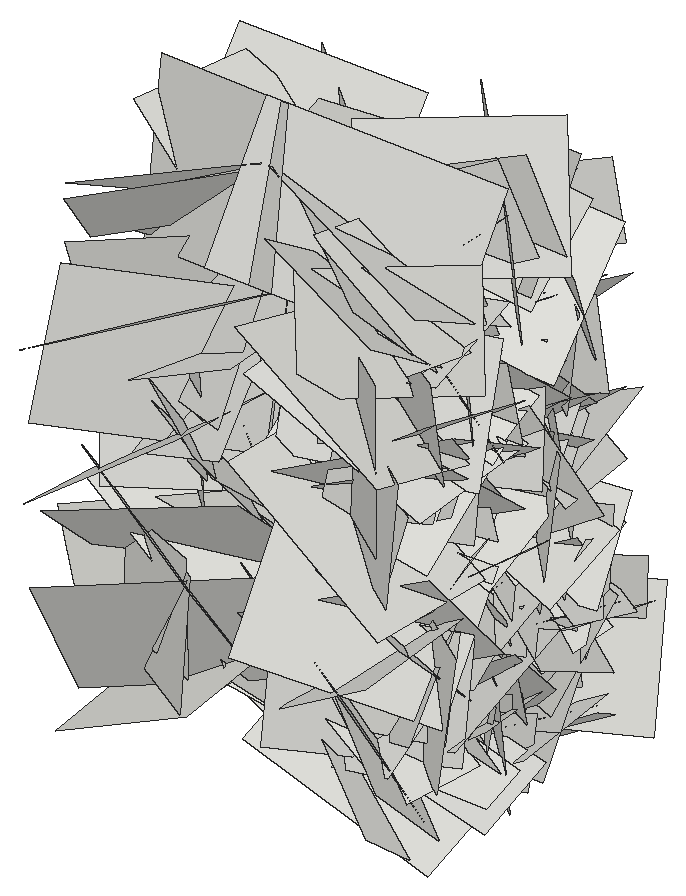
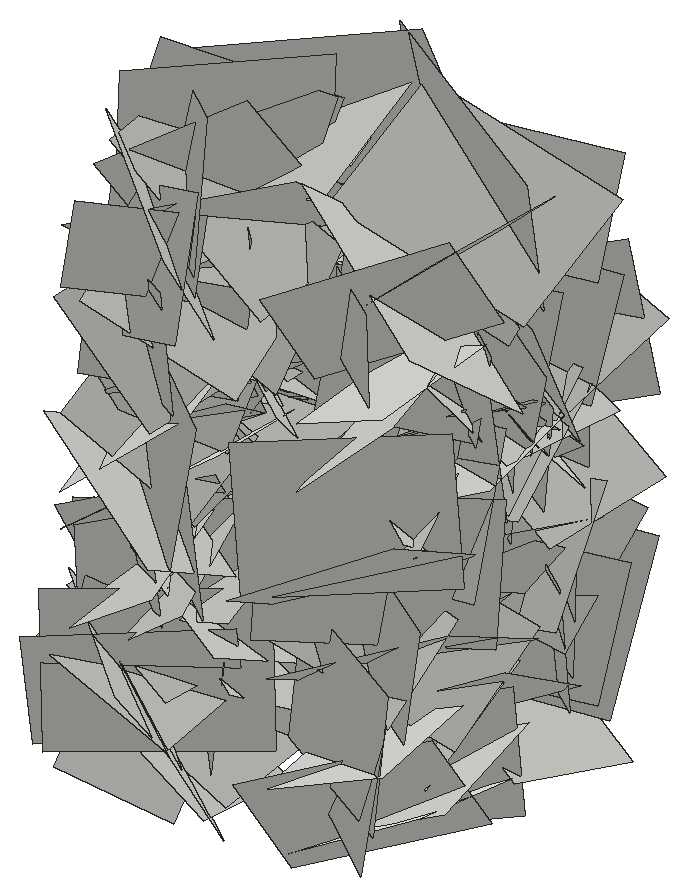
# SketchUp Ruby script. Lengths in inches.
U = 1.inch
M = Sketchup.active_model
def pt(a) = Geom::Point3d.new(a.map { |v| v * U })
def face(e, loops, mat)
  f = e.add_face(loops[0].map { |a| pt(a) })
  loops[1..].each { |l| e.add_face(l.map { |a| pt(a) }).erase! }
  f.material = f.back_material = mat if mat
  f
end
# faces: each face lists its corners as indices into pts; further lists are holes
def faces(e, pts, list, mat = nil) = list.each { |f| face(e, (f[0].is_a?(Array) ? f : [f]).map { |l| l.map { |i| pts[i] } }, mat) }
# xy, xz, yz: faces in a plane at the given z, y or x. An outline is a flat list of corners, or four numbers for a rectangle; further outlines are holes
def ring(l) = l.size == 4 ? [[l[0], l[1]], [l[2], l[1]], [l[2], l[3]], [l[0], l[3]]] : l.each_slice(2).to_a
def flat(e, list, mat, &to3) = list.each { |f| face(e, (f[0].is_a?(Array) ? f : [f]).map { |l| ring(l).map { |u, v| to3.(u, v) } }, mat) }
def xy(e, z, list, mat = nil) = flat(e, list, mat) { |x, y| [x, y, z] }
def xz(e, y, list, mat = nil) = flat(e, list, mat) { |x, z| [x, y, z] }
def yz(e, x, list, mat = nil) = flat(e, list, mat) { |y, z| [x, y, z] }
def lines(e, pts, list) = list.each { |a, b| e.add_line(pt(pts[a]), pt(pts[b])) }
# prism: a flat outline (further loops are holes) pulled along v
def prism(e, loops, v, mat = nil)
  f = face(e, loops, mat); d = Geom::Vector3d.new(v.map { |x| x * U })
  f.pushpull(f.normal.samedirection?(d) ? d.length : -d.length)
end
def box(e, o, s, mat = nil) = prism(e, [[o, [o[0] + s[0], o[1], o[2]], [o[0] + s[0], o[1] + s[1], o[2]], [o[0], o[1] + s[1], o[2]]]], [0, 0, s[2]], mat)
def at(x, y, z, deg = 0) = Geom::Transformation.translation(pt([x, y, z])) * Geom::Transformation.rotation(ORIGIN, Z_AXIS, deg.degrees)
def axes(o, x, y, z) = Geom::Transformation.new([*x, 0, *y, 0, *z, 0, *pt(o).to_a, 1])
def part(name) = M.definitions.add(name)
# library, detail: a bought-in or finely detailed component or shape, given as its bounding box
def library(name, o, s) = part(name).tap { |d| box(d.entities, o, s) }
def detail(e, o, s) = box(e.add_group.entities, o, s)
def put(e, d, t, mat = nil) = e.add_instance(d, t).tap { |i| i.material = mat if mat }
def group(e, t, mat = nil) = e.add_group.tap { |g| g.transformation = t; g.material = mat if mat }.entities
root = M.entities
c1 = part("Component\#6")
p = [[0.01,0,0],[0,3.24,4.54],[4.32,3.24,4.54],[4.33,0,0]]
faces(c1.entities,p,[[0,1,2,3]])
put(root,c1,axes([14.53,139.9,15.42],[0.08068,-0.00169,-0.87701],[0.08263,-0.87681,0.00845],[0.92595,0.07839,0.07566]))
put(root,c1,axes([18.5,139.99,14.29],[-0.01199,-0.16574,0.68191],[0.09091,0.67656,0.16586],[-0.73829,0.086,0.00935]))
put(root,c1,axes([18.5,147.58,14.43],[0.15626,-0.88067,0.15465],[0.14549,0.17716,0.87807],[-0.93656,-0.11942,0.1622]))
put(root,c1,axes([18.5,138.3,10.21],[0.07821,-0.14386,0.79141],[0.12147,0.78851,0.13265],[-0.84394,0.10016,0.09244]))
put(root,c1,axes([14.53,142.2,15.72],[-0.2001,0.61396,-1.10583],[-0.10306,-1.12181,-0.60624],[1.33676,0.00542,-0.21228]))
put(root,c1,axes([14.53,141.25,1.55],[0.11713,-0.0063,1.0149],[-0.13715,1.01248,0.02037],[1.06704,0.13083,-0.10878]))
put(root,c1,axes([14.53,144.34,6.82],[-0.01542,0.93301,-0.17325],[0.14993,-0.1692,-0.92309],[0.99466,0.03997,0.13646]))
put(root,c1,axes([14.53,137.99,14.66],[-0.08461,-0.27233,0.9902],[0.1352,0.98287,0.28059],[1.08015,-0.14435,0.04245]))
put(root,c1,axes([14.53,142.29,19.52],[0.02505,0.60517,0.90894],[-0.1077,0.90642,-0.60085],[1.15246,0.07156,-0.07591]))
put(root,c1,axes([14.53,144.58,9.97],[0.16827,0.58944,-0.69808],[-0.0398,-0.70373,-0.60275],[0.96765,-0.13145,0.0966]))
put(root,c1,axes([18.5,139.8125,20.98],[-0.02151,0.52563,-0.34386],[0.05265,-0.34162,-0.52514],[-0.66372,-0.04413,-0.03051]))
put(root,c1,axes([18.5,142.6,14.22],[0.18899,-0.6396,-0.42028],[-0.00285,-0.43205,0.65638],[-0.81124,-0.14749,-0.10022]))
put(root,c1,axes([18.5,145.36,10.15],[0.14636,-0.64891,0.3527],[0.01811,0.36152,0.65845],[-0.78267,-0.11298,0.08119]))
put(root,c1,axes([18.5,145.42,18.19],[0.07853,-0.05807,0.70782],[0.06912,0.70921,0.05136],[-0.74963,0.05931,0.07889]))
put(root,c1,axes([14.53,146.45,10.34],[0.10559,0.05407,-0.92917],[0.0532,-0.93343,-0.04894],[0.98516,0.04461,0.10223]))
put(root,c1,axes([18.5,141.95,12.73],[0.09992,0.55515,0.3498],[-0.02862,0.35638,-0.5583],[-0.69495,0.06514,0.07329]))
put(root,c1,axes([14.53,137.63,3.85],[-0.23328,-0.07655,1.22947],[0.08564,1.24535,0.092],[1.30295,-0.09556,0.21407]))
put(root,c1,axes([18.5,139.18,13.74],[0.11062,-0.13563,-0.63299],[-0.03095,-0.6415,0.13263],[-0.6855,0.00708,-0.10814]))
put(root,c1,axes([14.53,141.92,3.18],[0.02887,1.0089,0.10446],[0.06921,0.10254,-1.00735],[1.07292,-0.03376,0.06217]))
put(root,c1,axes([14.53,138.34,13.4],[0.1901,0.66514,0.65147],[-0.02496,0.66648,-0.67398],[0.98658,-0.1113,-0.14258]))
put(root,c1,axes([14.53,138.76,9.15],[0.08107,-0.07376,-0.93469],[0.12107,-0.93007,0.08274],[0.98644,0.12021,0.06666]))
put(root,c1,axes([14.53,139.52,8.83],[0.01584,-0.12995,-1.07448],[0.00128,-1.07458,0.12998],[1.14724,0.003,0.01469]))
put(root,c1,axes([14.53,137.41,10.49],[0.17918,0.96529,0.20208],[-0.06958,0.21558,-0.97489],[1.04307,-0.15144,-0.09975]))
put(root,c1,axes([14.53,141.07,4.77],[-0.0925,1.07709,-0.24358],[0.13853,-0.23255,-1.07513],[1.16232,0.11343,0.10875]))
put(root,c1,axes([14.53,143.54,11.83],[-0.01207,0.98557,0.48784],[0.03058,0.48797,-0.98515],[1.16528,-0.0026,0.03091]))
put(root,c1,axes([18.5,142.82,6.12],[-0.04161,-0.60559,-0.03198],[0.13563,-0.03959,0.59276],[-0.62835,0.03156,0.13006]))
put(root,c1,axes([14.53,142.72,8.07],[-0.13823,0.05764,1.30603],[-0.0986,1.30878,-0.06705],[1.38223,0.09912,0.12583]))
put(root,c1,axes([14.53,138.64,15.1],[-0.05154,1.07135,-0.23626],[0.10153,-0.23144,-1.06922],[1.15847,0.06794,0.08319]))
put(root,c1,axes([14.53,138.49,4.97],[-0.13436,1.04009,0.6085],[0.04809,0.61554,-1.04268],[1.27641,0.08629,0.10334]))
put(root,c1,axes([18.5,137.29,3.46],[0.14224,0.61257,0.15159],[-0.04066,0.16261,-0.62315],[-0.66768,0.1206,0.07024]))
put(root,c1,axes([14.53,137.21,11.6875],[-0.11385,0.72886,-0.88593],[0.14818,-0.87485,-0.7367],[1.20699,0.17615,0.00688]))
put(root,c1,axes([14.53,143.17,19.13],[0.20193,0.9279,-0.28366],[0.04691,-0.29708,-0.94209],[1.02744,-0.16881,0.09877]))
put(root,c1,axes([14.53,142.88,1.98],[0.0351,0.64216,0.95117],[0.00533,0.95147,-0.64254],[1.21649,-0.02269,-0.02463]))
put(root,c1,axes([14.53,137.64,18.89],[0.26376,-0.64139,0.69016],[0.02251,0.71746,0.65911],[0.99845,0.15326,-0.19718]))
put(root,c1,axes([14.53,140.93,18.6875],[-0.10901,-0.41314,-1.06231],[0.28274,-1.04573,0.38087],[1.17466,0.21337,-0.19026]))
put(root,c1,axes([14.53,141.75,2.91],[-0.11729,-1.19784,-0.30033],[0.11289,-0.30967,1.19584],[1.30414,-0.08092,-0.13053]))
put(root,c1,axes([14.53,143.08,17.68],[-0.06532,-0.13436,-1.17102],[0.13166,-1.16683,0.12734],[1.24247,0.11658,-0.07506]))
put(root,c1,axes([14.53,140.04,10.48],[-0.03722,-1.27767,0.05021],[-0.04996,0.05148,1.27723],[1.35446,-0.03321,0.04849]))
put(root,c1,axes([14.53,140.59,7.56],[-0.03383,1.06332,0.50099],[0.10932,0.50178,-1.05842],[1.24115,-0.01522,0.10688]))
put(root,c1,axes([14.53,137.94,15.45],[-0.03401,0.89045,-0.73196],[0.17038,-0.72163,-0.88493],[1.2099,0.12665,0.10405]))
put(root,c1,axes([14.53,146.96,20.2],[-0.19126,-1.0536,-0.82739],[0.10265,-0.84293,1.05228],[1.41631,-0.08119,-0.188]))
put(root,c1,axes([14.53,139.77,22.87],[0.12093,1.26112,-0.05281],[-0.18505,-0.03675,-1.25475],[1.32509,-0.12022,-0.17041]))
put(root,c1,axes([14.53,139.44,14.86],[-0.04621,-1.16691,0.31838],[0.12643,0.31289,1.16311],[1.27589,-0.07327,-0.10372]))
put(root,c1,axes([14.53,141.48,7.17],[0.20337,0.82379,-0.77749],[-0.08888,-0.77608,-0.84298],[1.19742,-0.19752,0.06948]))
put(root,c1,axes([14.53,138.37,16.22],[0.07456,0.76169,-0.90937],[0.0504,-0.91204,-0.76025],[1.25638,-0.00862,0.08446]))
put(root,c1,axes([14.53,148.05,8.79],[0.07068,0.0827,-1.14811],[0.1221,-1.14474,-0.07576],[1.21402,0.11031,0.07447]))
put(root,c1,axes([14.53,144.3,10.94],[0.16969,-0.07735,1.18237],[-0.06112,1.19119,0.08573],[1.2545,0.0685,-0.15576]))
put(root,c1,axes([14.53,144.73,5.33],[0.04426,-1.02294,0.56209],[0.16257,0.56238,1.01208],[1.2265,-0.03763,-0.15444]))
put(root,c1,axes([14.53,141.11,14.91],[0.10517,-0.78429,-0.79452],[0.18451,-0.77703,0.78876],[1.16892,0.19321,-0.05302]))
put(root,c1,axes([14.53,134.59,13.6],[0.14779,0.17555,1.29716],[-0.16453,1.29751,-0.15892],[1.37773,0.13612,-0.15813]))
put(root,c1,axes([14.53,148.13,7.79],[0.13698,0.11741,-1.23467],[-0.05668,-1.23967,-0.12348],[1.31343,-0.06574,0.12344]))
put(root,c1,axes([14.53,139.3125,6.46],[-0.05297,-0.89114,0.82127],[0.332,0.78454,0.87035],[1.24093,-0.24794,-0.1978]))
put(root,c1,axes([14.53,142.16,14.375],[-0.02255,-1.26636,-0.09652],[0.2141,-0.09868,1.25016],[1.3291,-0.00559,-0.20302]))
put(root,c1,axes([14.53,141.32,18.93],[-0.00931,-1.12138,0.55372],[0.26786,0.54072,1.09906],[1.29833,-0.1196,-0.22278]))
put(root,c1,axes([14.53,140.96,14.21],[0.1647,-0.56811,1.02456],[0.16232,1.03452,0.5504],[1.23116,-0.0604,-0.20963]))
put(root,c1,axes([14.53,137.06,3.09],[0.11239,-0.69918,1.17187],[0.18512,1.17269,0.68387],[1.43458,-0.09655,-0.18006]))
put(root,c1,axes([14.53,141.18,23.91],[0.20239,-0.45291,-1.29893],[0.24414,-1.28235,0.48098],[1.43758,0.28153,0.10118]))
put(root,c1,axes([28.31,141.18,23.91],[-0.20239,-0.45291,-1.29893],[-0.24414,-1.28235,0.48098],[-1.43758,0.28153,0.10118]))
put(root,c1,axes([28.31,137.06,3.09],[-0.11239,-0.69918,1.17187],[-0.18512,1.17269,0.68387],[-1.43458,-0.09655,-0.18006]))
put(root,c1,axes([28.31,140.96,14.21],[-0.1647,-0.56811,1.02456],[-0.16232,1.03452,0.5504],[-1.23116,-0.0604,-0.20963]))
put(root,c1,axes([28.31,141.32,18.93],[0.00931,-1.12138,0.55372],[-0.26786,0.54072,1.09906],[-1.29833,-0.1196,-0.22278]))
put(root,c1,axes([28.31,142.16,14.375],[0.02255,-1.26636,-0.09652],[-0.2141,-0.09868,1.25016],[-1.3291,-0.00559,-0.20302]))
put(root,c1,axes([28.31,139.3125,6.46],[0.05297,-0.89114,0.82127],[-0.332,0.78454,0.87035],[-1.24093,-0.24794,-0.1978]))
put(root,c1,axes([28.31,148.13,7.79],[-0.13698,0.11741,-1.23467],[0.05668,-1.23967,-0.12348],[-1.31343,-0.06574,0.12344]))
put(root,c1,axes([28.31,134.59,13.6],[-0.14779,0.17555,1.29716],[0.16453,1.29751,-0.15892],[-1.37773,0.13612,-0.15813]))
put(root,c1,axes([28.31,141.11,14.91],[-0.10517,-0.78429,-0.79452],[-0.18451,-0.77703,0.78876],[-1.16892,0.19321,-0.05302]))
put(root,c1,axes([28.31,144.73,5.33],[-0.04426,-1.02294,0.56209],[-0.16257,0.56238,1.01208],[-1.2265,-0.03763,-0.15444]))
put(root,c1,axes([28.31,144.3,10.94],[-0.16969,-0.07735,1.18237],[0.06112,1.19119,0.08573],[-1.2545,0.0685,-0.15576]))
put(root,c1,axes([28.31,138.37,16.22],[-0.07456,0.76169,-0.90937],[-0.0504,-0.91204,-0.76025],[-1.25638,-0.00862,0.08446]))
put(root,c1,axes([28.31,141.48,7.17],[-0.20337,0.82379,-0.77749],[0.08888,-0.77608,-0.84298],[-1.19742,-0.19752,0.06948]))
put(root,c1,axes([28.31,139.44,14.86],[0.04621,-1.16691,0.31838],[-0.12643,0.31289,1.16311],[-1.27589,-0.07327,-0.10372]))
put(root,c1,axes([28.31,139.77,22.87],[-0.12093,1.26112,-0.05281],[0.18505,-0.03675,-1.25475],[-1.32509,-0.12022,-0.17041]))
put(root,c1,axes([28.31,146.96,20.2],[0.19126,-1.0536,-0.82739],[-0.10265,-0.84293,1.05228],[-1.41631,-0.08119,-0.188]))
put(root,c1,axes([28.31,137.94,15.45],[0.03401,0.89045,-0.73196],[-0.17038,-0.72163,-0.88493],[-1.2099,0.12665,0.10405]))
put(root,c1,axes([28.31,140.59,7.56],[0.03383,1.06332,0.50099],[-0.10932,0.50178,-1.05842],[-1.24115,-0.01522,0.10688]))
put(root,c1,axes([28.31,140.04,10.48],[0.03722,-1.27767,0.05021],[0.04996,0.05148,1.27723],[-1.35446,-0.03321,0.04849]))
put(root,c1,axes([28.31,143.08,17.68],[0.06532,-0.13436,-1.17102],[-0.13166,-1.16683,0.12734],[-1.24247,0.11658,-0.07506]))
put(root,c1,axes([28.31,141.75,2.91],[0.11729,-1.19784,-0.30033],[-0.11289,-0.30967,1.19584],[-1.30414,-0.08092,-0.13053]))
put(root,c1,axes([28.31,140.93,18.6875],[0.10901,-0.41314,-1.06231],[-0.28274,-1.04573,0.38087],[-1.17466,0.21337,-0.19026]))
put(root,c1,axes([28.31,137.64,18.89],[-0.26376,-0.64139,0.69016],[-0.02251,0.71746,0.65911],[-0.99845,0.15326,-0.19718]))
put(root,c1,axes([28.31,142.88,1.98],[-0.0351,0.64216,0.95117],[-0.00533,0.95147,-0.64254],[-1.21649,-0.02269,-0.02463]))
put(root,c1,axes([28.31,143.17,19.13],[-0.20193,0.9279,-0.28366],[-0.04691,-0.29708,-0.94209],[-1.02744,-0.16881,0.09877]))
put(root,c1,axes([28.31,137.21,11.6875],[0.11385,0.72886,-0.88593],[-0.14818,-0.87485,-0.7367],[-1.20699,0.17615,0.00688]))
put(root,c1,axes([24.34,137.29,3.46],[-0.14224,0.61257,0.15159],[0.04066,0.16261,-0.62315],[0.66768,0.1206,0.07024]))
put(root,c1,axes([28.31,138.49,4.97],[0.13436,1.04009,0.6085],[-0.04809,0.61554,-1.04268],[-1.27641,0.08629,0.10334]))
put(root,c1,axes([28.31,138.64,15.1],[0.05154,1.07135,-0.23626],[-0.10153,-0.23144,-1.06922],[-1.15847,0.06794,0.08319]))
put(root,c1,axes([28.31,142.72,8.07],[0.13823,0.05764,1.30603],[0.0986,1.30878,-0.06705],[-1.38223,0.09912,0.12583]))
put(root,c1,axes([24.34,142.82,6.12],[0.04161,-0.60559,-0.03198],[-0.13563,-0.03959,0.59276],[0.62835,0.03156,0.13006]))
put(root,c1,axes([28.31,143.54,11.83],[0.01207,0.98557,0.48784],[-0.03058,0.48797,-0.98515],[-1.16528,-0.0026,0.03091]))
put(root,c1,axes([28.31,141.07,4.77],[0.0925,1.07709,-0.24358],[-0.13853,-0.23255,-1.07513],[-1.16232,0.11343,0.10875]))
put(root,c1,axes([28.31,137.41,10.49],[-0.17918,0.96529,0.20208],[0.06958,0.21558,-0.97489],[-1.04307,-0.15144,-0.09975]))
put(root,c1,axes([28.31,139.52,8.83],[-0.01584,-0.12995,-1.07448],[-0.00128,-1.07458,0.12998],[-1.14724,0.003,0.01469]))
put(root,c1,axes([28.31,138.76,9.15],[-0.08107,-0.07376,-0.93469],[-0.12107,-0.93007,0.08274],[-0.98644,0.12021,0.06666]))
put(root,c1,axes([28.31,138.34,13.4],[-0.1901,0.66514,0.65147],[0.02496,0.66648,-0.67398],[-0.98658,-0.1113,-0.14258]))
put(root,c1,axes([28.31,141.92,3.18],[-0.02887,1.0089,0.10446],[-0.06921,0.10254,-1.00735],[-1.07292,-0.03376,0.06217]))
put(root,c1,axes([24.34,139.18,13.74],[-0.11062,-0.13563,-0.63299],[0.03095,-0.6415,0.13263],[0.6855,0.00708,-0.10814]))
put(root,c1,axes([28.31,137.89,18.97],[-0.02244,-0.79516,0.48934],[-0.22215,0.48102,0.77258],[-0.96443,-0.0923,-0.18934]))
put(root,c1,axes([28.31,137.63,3.85],[0.23328,-0.07655,1.22947],[-0.08564,1.24535,0.092],[-1.30295,-0.09556,0.21407]))
put(root,c1,axes([24.34,141.95,12.73],[-0.09992,0.55515,0.3498],[0.02862,0.35638,-0.5583],[0.69495,0.06514,0.07329]))
put(root,c1,axes([28.31,146.45,10.34],[-0.10559,0.05407,-0.92917],[-0.0532,-0.93343,-0.04894],[-0.98516,0.04461,0.10223]))
put(root,c1,axes([24.34,145.42,18.19],[-0.07853,-0.05807,0.70782],[-0.06912,0.70921,0.05136],[0.74963,0.05931,0.07889]))
put(root,c1,axes([24.34,145.36,10.15],[-0.14636,-0.64891,0.3527],[-0.01811,0.36152,0.65845],[0.78267,-0.11298,0.08119]))
put(root,c1,axes([24.34,142.6,14.22],[-0.18899,-0.6396,-0.42028],[0.00285,-0.43205,0.65638],[0.81124,-0.14749,-0.10022]))
put(root,c1,axes([24.34,139.8125,20.98],[0.02151,0.52563,-0.34386],[-0.05265,-0.34162,-0.52514],[0.66372,-0.04413,-0.03051]))
put(root,c1,axes([28.31,144.58,9.97],[-0.16827,0.58944,-0.69808],[0.0398,-0.70373,-0.60275],[-0.96765,-0.13145,0.0966]))
put(root,c1,axes([28.31,142.29,19.52],[-0.02505,0.60517,0.90894],[0.1077,0.90642,-0.60085],[-1.15246,0.07156,-0.07591]))
put(root,c1,axes([28.31,137.99,14.66],[0.08461,-0.27233,0.9902],[-0.1352,0.98287,0.28059],[-1.08015,-0.14435,0.04245]))
put(root,c1,axes([28.31,144.34,6.82],[0.01542,0.93301,-0.17325],[-0.14993,-0.1692,-0.92309],[-0.99466,0.03997,0.13646]))
put(root,c1,axes([28.31,141.25,1.55],[-0.11713,-0.0063,1.0149],[0.13715,1.01248,0.02037],[-1.06704,0.13083,-0.10878]))
put(root,c1,axes([28.31,142.2,15.72],[0.2001,0.61396,-1.10583],[0.10306,-1.12181,-0.60624],[-1.33676,0.00542,-0.21228]))
put(root,c1,axes([24.34,138.3,10.21],[-0.07821,-0.14386,0.79141],[-0.12147,0.78851,0.13265],[0.84394,0.10016,0.09244]))
put(root,c1,axes([24.34,147.58,14.43],[-0.15626,-0.88067,0.15465],[-0.14549,0.17716,0.87807],[0.93656,-0.11942,0.1622]))
put(root,c1,axes([24.34,139.99,14.29],[0.01199,-0.16574,0.68191],[-0.09091,0.67656,0.16586],[0.73829,0.086,0.00935]))
put(root,c1,axes([28.31,139.9,15.42],[-0.08068,-0.00169,-0.87701],[-0.08263,-0.87681,0.00845],[-0.92595,0.07839,0.07566]))
put(root,c1,axes([24.34,145.32,5.58],[0.01721,-0.24816,-0.73855],[-0.187,-0.7207,0.23828],[0.80443,-0.16223,0.07119]))
put(root,c1,axes([28.31,140.66,10.67],[0.05387,-0.70807,-1.02445],[0.25854,-0.99979,0.70312],[-1.29449,-0.22915,0.09779]))
put(root,c1,axes([28.31,141.11,17.69],[-0.01651,0.23078,-0.87547],[-0.12637,-0.8685,-0.22682],[-0.95135,0.11136,0.04532]))
put(root,c1,axes([24.34,138.56,10.4375],[-0.05239,0.37979,0.51244],[0.10197,0.51253,-0.37059],[0.66837,-0.04842,0.0967]))
put(root,c1,axes([28.31,149.05,6.52],[0.16475,-0.3536,-1.09271],[0.00842,-1.10231,0.35784],[-1.21738,-0.05548,-0.1454]))
put(root,c1,axes([28.31,142.09,4.39],[-0.13266,-0.06807,0.83796],[-0.05074,0.84639,0.06161],[-0.88972,-0.03812,-0.12846]))
put(root,c1,axes([28.31,136.25,6.15],[-0.02753,0.62765,0.83331],[0.11118,0.83092,-0.62258],[-1.10023,0.06826,-0.08377]))
put(root,c1,axes([24.34,141.82,12.65],[0.04235,0.31596,0.66399],[-0.14644,0.65635,-0.30401],[0.76557,0.10807,-0.09488]))
put(root,c1,axes([28.31,145.41,21.68],[-0.17174,-0.50133,-0.77339],[0.12403,-0.79008,0.48764],[-0.96905,-0.01227,0.19948]))
put(root,c1,axes([24.34,139.97,19.34],[-0.20036,-0.21311,0.82685],[-0.01235,0.84743,0.21575],[0.90502,-0.03562,0.186]))
put(root,c1,axes([28.31,135.11,11.54],[0.10699,0.00448,1.06975],[-0.01257,1.07444,-0.00338],[-1.13388,-0.01149,0.10098]))
put(root,c1,axes([24.34,141.75,2.2],[0.07408,-0.19814,0.56205],[0.01701,0.56632,0.19765],[0.63148,0.00798,-0.07126]))
put(root,c1,axes([28.31,137.79,2.1],[0.03475,-0.78477,0.75119],[0.11687,0.75006,0.77877],[-1.14558,0.05272,0.10224]))
put(root,c1,axes([24.34,139.2,5.38],[-0.02645,-0.5119,-0.36479],[0.13209,-0.36186,0.49927],[0.65307,0.05245,-0.11575]))
put(root,c1,axes([28.31,139.48,6.78],[-0.1397,0.74364,0.31774],[-0.04551,0.31504,-0.75514],[-0.85599,-0.13812,-0.01171]))
put(root,c1,axes([28.31,146.4375,4.35],[0.18242,-1.06895,0.55133],[0.10581,0.56772,1.06956],[-1.27052,-0.1062,0.16823]))
put(root,c1,axes([24.34,141.96,13.08],[0.07799,-0.57044,-0.33182],[-0.05167,-0.33766,0.56968],[0.69762,0.03877,0.07929]))
put(root,c1,axes([28.31,137.55,18.4],[0.05522,0.7917,0.38208],[-0.20111,0.38385,-0.76951],[-0.90986,-0.0368,0.19328]))
put(root,c1,axes([24.34,140.67,1.375],[0.09858,-0.02009,0.69473],[-0.09996,0.69407,0.03269],[0.72991,0.09776,-0.08935]))
put(root,c1,axes([24.34,143.63,3.63],[0.04495,-0.13338,0.65571],[0.00407,0.65706,0.13341],[0.70927,0.00468,-0.04233]))
put(root,c1,axes([24.34,139.35,17.19],[0.06054,-0.33637,0.61942],[-0.0607,0.61718,0.34043],[0.74468,0.07766,-0.02261]))
put(root,c1,axes([28.31,145.52,15.88],[0.20612,-0.51117,0.96001],[-0.04532,0.97089,0.52562],[-1.15198,-0.12966,0.1511]))
put(root,c1,axes([24.34,136.74,12.93],[0.11437,0.04247,0.59628],[0.02624,0.60507,-0.04758],[0.63311,-0.03275,-0.10574]))
put(root,c1,axes([24.34,142.73,15.75],[-0.26089,1.021,-0.12695],[-0.10549,-0.15355,-1.04195],[1.08548,0.23047,-0.13178]))
put(root,c1,axes([28.31,139.41,15.5],[-0.07329,-0.02436,0.98546],[0.16551,0.97513,0.03506],[-1.03171,0.15816,-0.06438]))
put(root,c1,axes([24.34,143.53,7.33],[-0.11895,-0.88372,0.009],[-0.0734,0.01784,0.88799],[0.93392,-0.11115,0.07094]))
put(root,c1,axes([28.31,142.07,24.73],[0.13514,0.30002,-0.93652],[-0.09595,-0.93677,-0.31242],[-1.03799,0.12565,-0.09305]))
put(root,c1,axes([24.34,138.58,20.36],[-0.30182,0.3301,1.08442],[-0.18064,1.09293,-0.37743],[1.1879,0.25007,0.21813]))
put(root,c1,axes([28.31,143.76,15.19],[-0.09057,0.86782,-0.29614],[0.1091,-0.28647,-0.86917],[-0.96584,-0.11373,-0.07041]))
put(root,c1,axes([28.31,139.77,3.95],[-0.11908,-0.78329,-0.0515],[-0.03618,-0.0471,0.79084],[-0.83129,0.11425,-0.02704]))
put(root,c1,axes([24.34,146.8125,4.55],[-0.17148,-0.83232,0.10491],[0.08015,0.09194,0.84603],[0.88562,-0.16948,-0.05625]))
put(root,c1,axes([28.31,145.52,18.22],[0.02537,0.1253,-0.85934],[-0.08829,-0.85537,-0.12704],[-0.91628,0.08589,-0.01155]))
put(root,c1,axes([28.31,143.66,16.18],[-0.1105,0.58717,-0.52568],[-0.01323,-0.53143,-0.59111],[-0.83529,-0.06926,0.0789]))
put(root,c1,axes([28.31,147.01,9.44],[0.18802,-1.10018,-0.17062],[0.06994,-0.16208,1.11371],[-1.17806,-0.18521,0.03889]))
put(root,c1,axes([24.34,143.33,2.25],[0.06381,-0.71847,0.0034],[-0.02834,0.00117,0.7205],[0.76106,0.06028,0.02655]))
put(root,c1,axes([28.31,144.05,16.5],[-0.02895,-0.76847,-0.41691],[0.01722,-0.41749,0.76847],[-0.92657,0.01625,0.02731]))
put(root,c1,axes([28.31,143.95,11.7],[0.02215,-0.88691,-0.38082],[0.08723,-0.37788,0.88459],[-1.0194,-0.05161,0.06742]))
put(root,c1,axes([24.34,147.56,10.64],[0.00206,-0.13591,-0.77504],[-0.03252,-0.77447,0.13573],[0.83344,-0.02988,0.00721]))
put(root,c1,axes([24.34,142.57,12.97],[-0.12959,-0.66136,0.5647],[0.03976,0.56572,0.67067],[0.92097,-0.11748,0.0505]))
put(root,c1,axes([28.31,141.85,18.04],[0.12661,-0.3078,1.12748],[0.24587,1.11705,0.28038],[-1.21422,0.1941,0.17434]))
put(root,c1,axes([24.34,147.06,19.23],[-0.16196,0.05609,-0.92604],[0.00217,-0.93849,-0.05718],[0.9834,0.01131,-0.15239]))
put(root,c1,axes([24.34,141.5625,11.54],[-0.13399,-0.80117,0.38482],[0.02481,0.38556,0.81039],[0.9418,-0.12414,0.0334]))
put(root,c1,axes([24.34,149.3125,5.88],[-0.15882,-0.57412,-0.80425],[-0.08368,-0.80389,0.58857],[1.04409,-0.15176,-0.07517]))
put(root,c1,axes([28.31,143.03,2.65],[0.18528,-0.93043,-0.12384],[-0.14778,-0.15031,0.9325],[-0.98392,-0.15263,-0.16338]))
put(root,c1,axes([24.34,141.35,5.69],[0.05421,0.52298,-0.48745],[0.04158,-0.49001,-0.52162],[0.75668,-0.01054,0.06359]))
put(root,c1,axes([28.31,145.65,3.28],[-0.1646,0.60158,-0.34623],[-0.0091,-0.35642,-0.61544],[-0.73568,-0.13018,0.08507]))
put(root,c1,axes([24.34,139.62,7.21],[-0.15609,-0.9187,-0.23757],[-0.00588,-0.23958,0.92989],[1.00583,-0.14396,-0.03143]))
put(root,c1,axes([24.34,143.17,8.1],[0.04482,0.75985,0.07181],[0.00358,0.07173,-0.76102],[0.80902,-0.04241,-0.00061]))
put(root,c1,axes([24.34,141.47,13.3125],[-0.15098,-0.93805,0.13539],[-0.00567,0.13771,0.94846],[1.00463,-0.1402,0.0257]))
put(root,c1,axes([28.31,139.94,18.75],[0.02341,-0.9115,0.17831],[0.09444,0.17962,0.90714],[-0.97996,-0.00447,0.09169]))
put(root,c1,axes([24.34,144.39,10.35],[-0.12238,0.87118,-0.30871],[-0.00416,-0.31157,-0.87778],[0.97971,0.1075,-0.04229]))
put(root,c1,axes([24.34,135.6875,17.375],[-0.11773,0.10526,0.9962],[-0.108,0.99592,-0.11659],[1.05635,0.11356,0.09911]))
put(root,c1,axes([24.34,136.7,5.12],[0.11008,0.58852,-0.4619],[-0.03608,-0.46213,-0.59646],[0.7922,-0.10282,0.03702]))
put(root,c1,axes([28.31,147.32,10.4375],[0.06119,-0.47987,-0.75245],[0.01649,-0.75336,0.48165],[-0.94584,-0.04418,-0.04028]))
